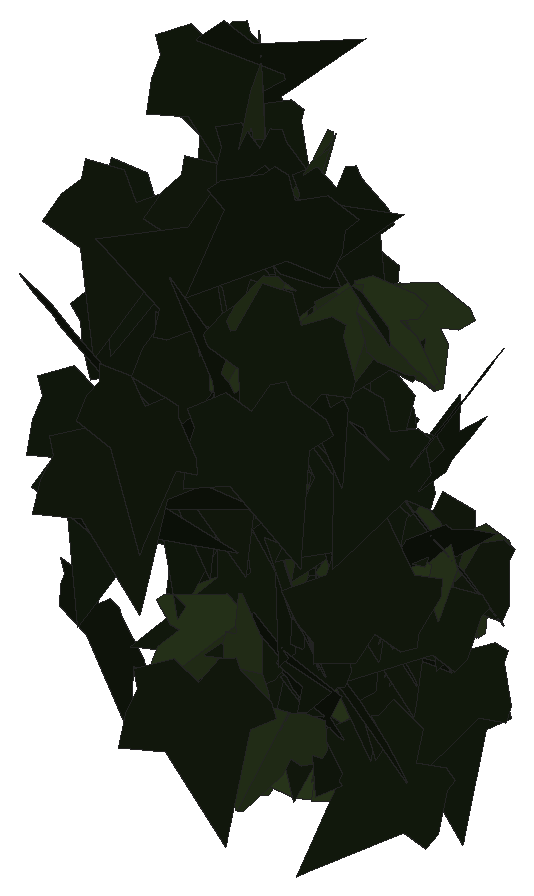
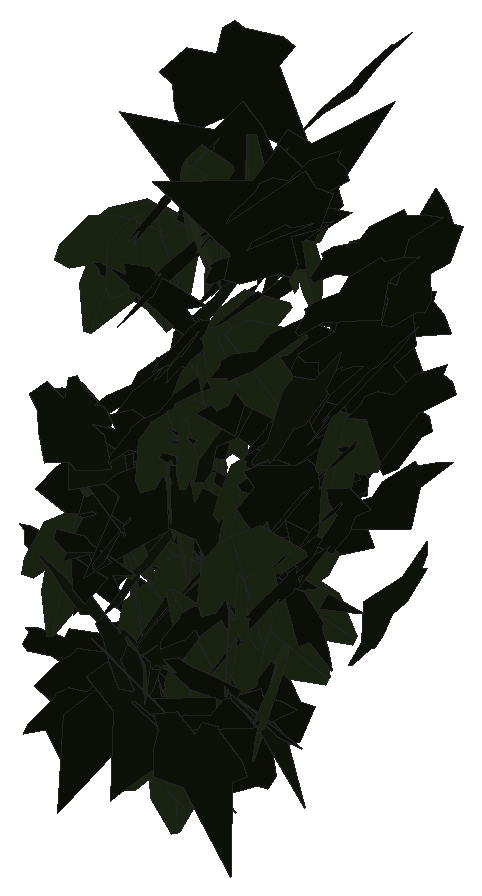
# SketchUp Ruby script. Lengths in inches.
U = 1.inch
M = Sketchup.active_model
def pt(a) = Geom::Point3d.new(a.map { |v| v * U })
def face(e, loops, mat)
  f = e.add_face(loops[0].map { |a| pt(a) })
  loops[1..].each { |l| e.add_face(l.map { |a| pt(a) }).erase! }
  f.material = f.back_material = mat if mat
  f
end
# faces: each face lists its corners as indices into pts; further lists are holes
def faces(e, pts, list, mat = nil) = list.each { |f| face(e, (f[0].is_a?(Array) ? f : [f]).map { |l| l.map { |i| pts[i] } }, mat) }
# xy, xz, yz: faces in a plane at the given z, y or x. An outline is a flat list of corners, or four numbers for a rectangle; further outlines are holes
def ring(l) = l.size == 4 ? [[l[0], l[1]], [l[2], l[1]], [l[2], l[3]], [l[0], l[3]]] : l.each_slice(2).to_a
def flat(e, list, mat, &to3) = list.each { |f| face(e, (f[0].is_a?(Array) ? f : [f]).map { |l| ring(l).map { |u, v| to3.(u, v) } }, mat) }
def xy(e, z, list, mat = nil) = flat(e, list, mat) { |x, y| [x, y, z] }
def xz(e, y, list, mat = nil) = flat(e, list, mat) { |x, z| [x, y, z] }
def yz(e, x, list, mat = nil) = flat(e, list, mat) { |y, z| [x, y, z] }
def lines(e, pts, list) = list.each { |a, b| e.add_line(pt(pts[a]), pt(pts[b])) }
# prism: a flat outline (further loops are holes) pulled along v
def prism(e, loops, v, mat = nil)
  f = face(e, loops, mat); d = Geom::Vector3d.new(v.map { |x| x * U })
  f.pushpull(f.normal.samedirection?(d) ? d.length : -d.length)
end
def box(e, o, s, mat = nil) = prism(e, [[o, [o[0] + s[0], o[1], o[2]], [o[0] + s[0], o[1] + s[1], o[2]], [o[0], o[1] + s[1], o[2]]]], [0, 0, s[2]], mat)
def at(x, y, z, deg = 0) = Geom::Transformation.translation(pt([x, y, z])) * Geom::Transformation.rotation(ORIGIN, Z_AXIS, deg.degrees)
def axes(o, x, y, z) = Geom::Transformation.new([*x, 0, *y, 0, *z, 0, *pt(o).to_a, 1])
def part(name) = M.definitions.add(name)
# library, detail: a bought-in or finely detailed component or shape, given as its bounding box
def library(name, o, s) = part(name).tap { |d| box(d.entities, o, s) }
def detail(e, o, s) = box(e.add_group.entities, o, s)
def put(e, d, t, mat = nil) = e.add_instance(d, t).tap { |i| i.material = mat if mat }
def group(e, t, mat = nil) = e.add_group.tap { |g| g.transformation = t; g.material = mat if mat }.entities
root = M.entities
M.materials.add("efeu1").color = [18, 25, 13]
M.materials.add("efeu2").color = [43, 57, 29]
c1 = part("ivyleaf_9")
p = [[1.54,2.16,1.25],[1.36,2.04,1.19],[-0.21,0.99,0.68],[-0.71,1.11,0.82],[-0.85,0.86,0.67],[-0.8,0.17,0.21],
  [-0.9,-0.01,0.1],[-0.67,-0.16,-0.02],[-0.08,-0.08,-0.05],[-0.03,-0.6,-0.4],[0.65,-0.88,-0.66],[0.83,-0.6,-0.49],
  [1.29,-0.42,-0.43],[1.8125,-0.07,-0.26],[1.21,0.44,0.15]]
faces(c1.entities,p,[[0,1,2,3,4,5,6,7,8,9,10,11,12,13,14]],"efeu1")
c2 = part("ivyleaf_10")
p = [[0,0.5,-0.03],[-0.0625,2.02,-0.43],[-0.19,2.01,-0.46],[-0.54,1.05,-0.29],[-0.52,0.625,-0.18],[-0.83,0.76,-0.28],
  [-1.16,0.64,-0.33],[-1.15,0.33,-0.24],[-0.77,-0.39,0.02],[-0.3,-0.51,0.16],[0.04,-0.48,0.23],[-0.02,2.01,-0.4375],
  [-0.06,2.01,-0.43],[0.04,-0.49,0.23],[0.67,-0.49,0.14],[1.38,0.36,-0.2],[1.375,0.51,-0.24],[0.81,0.65,-0.19],
  [0.62,0.59,-0.15],[0.6,1.09,-0.28],[0.5,1.23,-0.31]]
faces(c2.entities,p,[[0,1,2,3,4,5,6,7,8,9,10],[11,12,0,13,14,15,16,17,18,19,20]],"efeu2")
put(root,c1,axes([37.96,220.71,244.54],[-0.12354,-0.47923,0.07127],[-0.01994,-0.06846,-0.49489],[0.48409,-0.12511,-0.00219]))
put(root,c1,axes([37.8125,220.9,246.18],[0.24494,-0.40918,-0.15026],[-0.026,0.15834,-0.47355],[0.43512,0.2398,0.05629]))
put(root,c1,axes([37.8,222.26,246.11],[0.03675,-0.38064,0.32212],[0.1316,-0.30414,-0.37441],[0.48097,0.1123,0.07783]))
put(root,c1,axes([37.99,221.21,247.15],[-0.13138,-0.47417,0.08886],[-0.01747,-0.08736,-0.492],[0.48211,-0.13239,0.00639]))
put(root,c2,axes([38.11,221.03,245.32],[0.02039,-0.43408,-0.2473],[0.04694,0.24808,-0.43157],[0.49737,-0.00562,0.05087]))
put(root,c1,axes([37.83,220.61,243.18],[0.15949,-0.4167,0.22567],[0.09762,-0.20411,-0.44588],[0.46372,0.18628,0.01625]))
put(root,c1,axes([37.97,220.39,245.57],[-0.00115,-0.46441,-0.18526],[-0.01173,0.18524,-0.46427],[0.49986,0.00328,-0.01132]))
put(root,c2,axes([38.11,222.14,243.03],[-0.24291,0.43502,0.04189],[-0.01309,0.04066,-0.49817],[-0.43684,-0.24311,-0.00837]))
put(root,c1,axes([38,222.02,244.15],[0.27996,-0.29232,-0.29354],[-0.10891,0.28989,-0.39256],[0.3997,0.28374,0.09864]))
put(root,c1,axes([38.15,220.7,247.46],[-0.16154,-0.47243,0.02683],[-0.00693,-0.02598,-0.49928],[0.47314,-0.16167,0.00184]))
put(root,c1,axes([38.61,221.9,242.54],[-0.24635,0.39084,0.19118],[-0.11648,0.15244,-0.46173],[-0.41922,-0.27203,0.01594]))
put(root,c1,axes([38.21,221.57,244.29],[-0.00683,-0.48185,0.13332],[-0.00552,-0.13325,-0.48188],[0.49992,-0.00806,-0.0035]))
put(root,c1,axes([38.21,221.82,248.625],[0.01018,-0.46344,-0.18739],[-0.01552,0.18705,-0.46344],[0.49966,0.01525,-0.01058]))
put(root,c1,axes([38.6,222.85,242.4],[-0.16091,0.47337,-0.00515],[-0.01155,-0.00937,-0.49978],[-0.47326,-0.16072,0.01395]))
put(root,c2,axes([38.47,222.3125,244.32],[-0.20958,-0.43661,0.12428],[-0.0076,-0.13349,-0.48179],[0.45389,-0.20384,0.04932]))
put(root,c1,axes([38.2,221.38,244.9],[0.12038,-0.48516,0.01118],[0.0025,-0.01089,-0.49988],[0.48529,0.12041,-0.0002]))
put(root,c1,axes([38.13,221.5,244.9],[0.07711,-0.16743,-0.46478],[0.16347,0.45255,-0.13591],[0.46619,-0.131,0.12454]))
put(root,c1,axes([38.4,222.22,247.93],[-0.22111,-0.43508,0.10872],[0.00428,-0.12325,-0.48455],[0.44843,-0.21335,0.05823]))
put(root,c1,axes([38.1,222.01,248.16],[0.135,-0.04118,0.47967],[0.47348,0.10152,-0.12454],[-0.08714,0.48785,0.06641]))
put(root,c1,axes([38.1,219.6875,246.69],[0.26349,-0.28862,0.31188],[0.24141,-0.20034,-0.38934],[0.34971,0.35576,0.03378]))
put(root,c1,axes([38.6,220.89,245.02],[0.07759,0.49379,0.01219],[0.00013,0.01232,-0.49985],[-0.49394,0.07757,0.00179]))
put(root,c1,axes([38.36,221.5625,243.68],[-0.25895,-0.06159,-0.42326],[0.42123,0.04914,-0.26486],[0.07422,-0.49375,0.02643]))
put(root,c2,axes([38.54,222.28,243.87],[0.33302,-0.33002,-0.17374],[0.0094,0.24028,-0.43838],[0.37284,0.28871,0.16624]))
put(root,c1,axes([38.44,221.37,245.73],[0.0045,-0.49777,0.04695],[0.00857,-0.04687,-0.49772],[0.49991,0.00528,0.00811]))
put(root,c2,axes([38.66,221.54,243.07],[-0.08305,-0.34895,0.34834],[-0.00646,-0.35245,-0.3546],[0.49301,-0.0634,0.05403]))
put(root,c1,axes([38.45,221.42,245.01],[-0.04855,-0.43972,-0.23299],[0.05216,0.22831,-0.44176],[0.4949,-0.0672,0.02371]))
put(root,c1,axes([38.39,221.94,242],[0.02494,-0.02361,0.49882],[0.43276,0.25024,-0.00979],[-0.24919,0.43223,0.03292]))
put(root,c1,axes([38.96,222.61,242.92],[-0.48833,0.00779,0.10709],[-0.10733,-0.049,-0.48588],[0.00293,-0.49753,0.04953]))
put(root,c1,axes([38.625,222.54,242.52],[-0.19659,-0.45499,-0.06582],[0.01532,0.06506,-0.49551],[0.45948,-0.19684,-0.01164]))
put(root,c2,axes([38.8,221.7,248.63],[0.20938,-0.3969,-0.22054],[-0.01736,0.23568,-0.44063],[0.45372,0.19217,0.08491]))
put(root,c2,axes([38.78,221.83,244.86],[0.0064,-0.42454,-0.26406],[0.053,0.26317,-0.42182],[0.49714,-0.02259,0.04838]))
put(root,c2,axes([38.8,220.95,247.44],[0.16531,-0.47023,0.03944],[0.00288,-0.04079,-0.49833],[0.47187,0.16498,-0.01078]))
put(root,c1,axes([38.71,221.7,246.42],[-0.10637,-0.48741,-0.03343],[0.00489,0.03315,-0.49888],[0.48853,-0.10646,-0.00229]))
put(root,c2,axes([39.01,220.98,243.19],[-0.16994,-0.24865,0.39912],[-0.17326,-0.36141,-0.29894],[0.43715,-0.2399,0.03667]))
put(root,c2,axes([38.96,221.72,246.31],[-0.27625,-0.30282,0.28634],[-0.08549,-0.29505,-0.39451],[0.4079,-0.26692,0.11123]))
put(root,c1,axes([38.5,219.62,245],[0.42498,0.07261,0.25321],[0.24958,0.04275,-0.43114],[-0.08426,0.49285,0.0001]))
put(root,c1,axes([38.72,222.37,243.74],[-0.07377,-0.49231,-0.04683],[-0.00314,0.04781,-0.4977],[0.49452,-0.07314,-0.01014]))
put(root,c2,axes([38.74,222.29,242.84],[-0.36885,-0.1766,0.28769],[0.2826,0.07151,0.40623],[-0.18462,0.46228,0.04706]))
put(root,c1,axes([38.83,220.875,245.25],[0.16335,0.06778,0.46768],[0.24664,0.40986,-0.14554],[-0.4031,0.27825,0.10047]))
put(root,c1,axes([38.88,221.26,247.53],[-0.14764,-0.4776,0.0099],[-0.00315,-0.00939,-0.4999],[0.4777,-0.14767,-0.00024]))
put(root,c1,axes([39.19,221.96,244.69],[-0.19029,0.46185,0.02205],[-0.00887,0.02019,-0.49951],[-0.46229,-0.1905,0.00051]))
put(root,c2,axes([39.07,222.33,242.83],[-0.0141,-0.46427,0.18509],[0.00949,-0.18537,-0.46427],[0.49971,-0.00958,0.01404]))
put(root,c2,axes([39.08,221.64,246.53],[-0.05554,-0.46368,0.17864],[-0.0036,-0.17937,-0.4667],[0.49689,-0.05313,0.01658]))
put(root,c2,axes([39.11,221.63,244.47],[-0.49558,0.06051,0.02725],[-0.02746,-0.00005,-0.49925],[-0.06042,-0.49632,0.00337]))
put(root,c1,axes([39.39,221.33,243.45],[-0.40865,-0.07336,0.27861],[-0.27547,-0.04216,-0.41514],[0.0844,-0.49279,-0.00595]))
put(root,c1,axes([38.72,219.57,245.33],[0.36132,0.01669,0.34521],[0.34323,0.04116,-0.36125],[-0.04048,0.49802,0.01828]))
put(root,c2,axes([39.13,222.6,242.03],[-0.33719,-0.36551,0.05199],[0.05232,-0.11701,-0.48329],[0.36546,-0.32049,0.11715]))
put(root,c2,axes([39.06,222.49,241.9375],[0.00063,-0.20372,0.45662],[0.15138,-0.43511,-0.19433],[0.47653,0.13849,0.06112]))
put(root,c1,axes([39.25,222.65,242.57],[0.1329,0.41844,0.23926],[-0.01403,0.25144,-0.43195],[-0.48181,0.1081,0.07858]))
put(root,c1,axes([39.08,219.28,245.79],[-0.18011,-0.37787,-0.27344],[0.12041,0.24552,-0.4186],[0.45062,-0.21664,0.00256]))
put(root,c1,axes([39.49,222.72,242.29],[-0.49723,0.04762,0.02221],[-0.02225,0.00054,-0.4995],[-0.04759,-0.49773,0.00158]))
put(root,c2,axes([39.61,220.66,243.12],[-0.14071,0.08535,0.47214],[-0.46858,0.08128,-0.15435],[-0.1031,-0.48591,0.05711]))
put(root,c2,axes([39.08,221.51,241.98],[-0.06346,-0.15771,-0.47021],[0.31319,0.35483,-0.16127],[0.38456,-0.315,0.05375]))
put(root,c1,axes([39.04,221.24,246.75],[0.20052,-0.40808,-0.20799],[0.00025,0.22715,-0.44543],[0.45803,0.17853,0.0913]))
put(root,c1,axes([39.0625,221.44,248.02],[0.17718,-0.4667,-0.0282],[-0.01039,0.02622,-0.4992],[0.46744,0.17749,-0.0004]))
put(root,c2,axes([39.34,221.88,245.26],[0.04598,-0.49435,-0.05921],[-0.01432,0.05812,-0.4964],[0.49768,0.04735,-0.00882]))
put(root,c1,axes([39.4375,220.26,247.34],[-0.01755,0.015,0.49947],[-0.38324,-0.32111,-0.00382],[0.32065,-0.38297,0.02277]))
put(root,c2,axes([39.3125,222.27,244.87],[0.18484,-0.46087,-0.05864],[0.00327,0.0644,-0.49582],[0.46457,0.18291,0.02682]))
put(root,c1,axes([39.16,222.01,243.44],[-0.00539,-0.36133,0.34556],[0.02843,-0.34524,-0.36055],[0.49916,0.01576,0.02427]))
put(root,c1,axes([39.72,221.5,242.78],[-0.31089,0.26856,0.285],[-0.22972,0.16962,-0.41043],[-0.31714,-0.38614,0.01792]))
put(root,c2,axes([39.44,222.14,245.37],[-0.19502,-0.43799,0.14189],[-0.00097,-0.1537,-0.47579],[0.4604,-0.18585,0.0591]))
put(root,c1,axes([39.31,221.93,242.74],[-0.14978,-0.47421,-0.05183],[0.0107,0.05098,-0.49728],[0.47692,-0.15008,-0.00513]))
put(root,c1,axes([39.25,221.22,247.13],[-0.02145,-0.47988,0.13877],[0.01731,-0.13953,-0.47983],[0.49924,-0.01578,0.0226]))
put(root,c2,axes([39.54,221.55,245.7],[-0.05461,-0.44926,0.21256],[-0.02241,-0.21139,-0.45256],[0.4965,-0.05896,0.00295]))
put(root,c2,axes([39.47,221.8,247.92],[0.25745,-0.41902,0.09023],[0.03341,-0.08532,-0.49153],[0.42732,0.25912,-0.01594]))
put(root,c1,axes([39.84,222.65,242.8125],[-0.44897,0.20698,0.07474],[-0.08281,-0.00159,-0.49309],[-0.20388,-0.45515,0.03571]))
put(root,c1,axes([39.19,221.82,245.22],[0.20396,-0.34625,0.29751],[0.23964,-0.19615,-0.39256],[0.38856,0.30272,0.08593]))
put(root,c1,axes([39.83,222.49,242.99],[-0.34022,0.36251,-0.05326],[0.0411,-0.03446,-0.49711],[-0.36409,-0.34263,-0.00636]))
put(root,c1,axes([39.31,222.53,242.95],[0.02599,-0.28604,0.40927],[0.23612,-0.35407,-0.26245],[0.43997,0.20691,0.11668]))
put(root,c2,axes([39.64,221.55,248.02],[0.13789,-0.47936,0.03459],[0.00452,-0.03469,-0.49877],[0.48059,0.13786,-0.00524]))
put(root,c1,axes([39.44,222.11,244.83],[0.02766,-0.21724,-0.44949],[0.02348,0.45025,-0.21616],[0.49868,-0.00915,0.03511]))
put(root,c1,axes([39.55,219.91,243.24],[-0.1136,-0.42264,-0.24181],[0.06184,0.23378,-0.43764],[0.48298,-0.12934,-0.00084]))
put(root,c2,axes([39.66,221.46,241.74],[0.30332,0.3785,-0.12138],[0.07387,0.09636,0.48504],[0.39056,-0.31218,0.00254]))
put(root,c2,axes([39.61,222.62,242.67],[-0.34873,0.28021,-0.22332],[0.14591,-0.17356,-0.44563],[-0.32726,-0.37598,0.03928]))
put(root,c2,axes([39.88,220.68,242.6],[-0.28797,-0.36641,0.18114],[-0.12022,-0.13586,-0.46593],[0.39067,-0.3119,-0.00985]))
put(root,c2,axes([39.8,221.99,243.33],[0.12952,0.4081,-0.25822],[-0.17497,-0.20953,-0.41891],[-0.45012,0.19888,0.08854]))
put(root,c2,axes([39.75,222.46,242.64],[0.2757,-0.3919,-0.14284],[0.00303,0.1731,-0.46907],[0.41711,0.25778,0.09782]))
put(root,c1,axes([39.84,220.07,246.31],[0.16086,-0.43233,0.19291],[-0.02603,0.19536,0.45952],[-0.4727,-0.15788,0.04034]))
put(root,c2,axes([39.81,220.69,246.99],[0.06862,0.34856,-0.35185],[-0.14786,-0.3246,-0.35039],[-0.47268,0.15214,0.05853]))
put(root,c1,axes([39.5625,221.46,247.375],[0.27395,-0.31436,-0.27592],[-0.06589,0.29328,-0.39956],[0.41305,0.25528,0.11926]))
put(root,c1,axes([39.625,222.15,245.58],[0.01672,-0.4997,0.00498],[-0.00584,-0.00518,-0.49994],[0.49969,0.01666,-0.00601]))
put(root,c1,axes([39.76,221.52,245.38],[0.42998,0.14103,-0.21266],[-0.20488,-0.05759,-0.45244],[-0.15211,0.47623,0.00826]))
put(root,c2,axes([39.83,221.91,242.11],[0.06883,-0.49116,-0.06344],[-0.00242,0.06372,-0.49592],[0.49523,0.06857,0.00639]))
put(root,c1,axes([39.6,222.5,243.875],[0.02038,-0.39437,0.30668],[0.06832,-0.30185,-0.3927],[0.49489,0.05791,0.04159]))
put(root,c1,axes([39.84,222.12,244.82],[-0.24684,-0.40581,0.15616],[-0.05281,-0.15026,-0.47396],[0.4316,-0.25048,0.03131]))
put(root,c1,axes([39.65,221.3,246.25],[0.12972,-0.45072,-0.17327],[-0.03994,0.16878,-0.46895],[0.48123,0.13551,0.00779]))
put(root,c2,axes([39.87,220.93,244.0625],[-0.2967,0.39444,0.07988],[-0.05214,0.06073,-0.49355],[-0.39906,-0.30121,0.00509]))
put(root,c1,axes([39.53,221.27,242.76],[0.00922,-0.18967,0.46254],[0.31086,-0.36012,-0.15387],[0.39151,0.29041,0.11128]))
put(root,c1,axes([39.64,221.875,243.25],[0.14674,-0.47709,0.02922],[0.01095,-0.02721,-0.49914],[0.47786,0.14712,0.00246]))
put(root,c1,axes([39.72,221.97,242.1],[-0.12568,-0.35642,0.32736],[0.10145,-0.35011,-0.34224],[0.4732,-0.01961,0.16032]))
put(root,c1,axes([40.14,222.14,245.17],[-0.47695,-0.13296,0.06961],[-0.06893,-0.01195,-0.49508],[0.13331,-0.48185,-0.00693]))
put(root,c1,axes([40.03,222,244.53],[-0.41555,-0.2677,-0.07521],[0.05499,0.05346,-0.49408],[0.27258,-0.4189,-0.01499]))
put(root,c1,axes([39.72,221.375,246.23],[0.15292,-0.45106,0.15218],[0.06816,-0.13745,-0.47588],[0.47114,0.16628,0.01945]))
put(root,c1,axes([39.79,222.34,242.74],[-0.03892,-0.44839,0.21779],[0.12369,-0.2203,-0.43147],[0.48289,0.02029,0.12807]))
put(root,c1,axes([39.95,222.5,242.45],[0.43859,0.19029,-0.1464],[-0.1401,-0.04475,-0.47788],[-0.19497,0.4602,0.01406]))
put(root,c1,axes([40.05,221.85,244.69],[-0.24328,-0.29715,0.32019],[-0.06607,-0.33725,-0.36318],[0.4318,-0.21902,0.12483]))
put(root,c1,axes([40.4,220.99,243.52],[-0.31732,0.31233,0.22751],[-0.18321,0.13759,-0.44441],[-0.34021,-0.36541,0.02712]))
put(root,c1,axes([39.67,220.8125,247.62],[0.08703,-0.04141,0.49062],[0.47981,-0.10467,-0.09395],[0.11048,0.48717,0.02152]))
put(root,c1,axes([39.8,221.84,244.04],[0.30123,-0.39907,0.00244],[-0.0004,-0.00336,-0.49999],[0.39908,0.30122,-0.00234]))
put(root,c2,axes([40.08,222.08,243.6],[0.29961,-0.39857,-0.03706],[0.00486,0.04991,-0.49748],[0.40026,0.29774,0.03378]))
put(root,c1,axes([39.78,221.49,243.03],[0.34883,-0.33811,0.11832],[0.08525,-0.08206,-0.4858],[0.34793,0.35909,0.0004]))
put(root,c1,axes([39.92,221.5,247.87],[0.20293,-0.45089,-0.07429],[-0.02371,0.07079,-0.4944],[0.45635,0.20418,0.00735]))
put(root,c2,axes([40.32,221.71,243.98],[0.27863,0.28788,-0.29916],[-0.27391,-0.14329,-0.39299],[-0.312,0.38288,0.07786]))
put(root,c1,axes([40.33,221.76,246.75],[-0.4809,-0.12808,-0.04832],[0.05269,-0.01029,-0.49711],[0.12635,-0.48321,0.0234]))
put(root,c1,axes([40.1875,220.57,246.9375],[-0.28061,-0.41321,-0.02279],[0.01512,0.01729,-0.49947],[0.41356,-0.281,0.00279]))
put(root,c1,axes([40.46,220.13,248.5625],[0.04692,0.17453,-0.4662],[-0.16609,-0.43594,-0.17992],[-0.46927,0.17175,0.01706]))
put(root,c2,axes([40.54,222.03,244.17],[0.31667,-0.10286,-0.37302],[-0.34681,0.13831,-0.33256],[0.17159,0.46935,0.01625]))
put(root,c1,axes([40.14,221.84,243.96],[-0.00916,-0.46801,-0.17574],[0.03931,0.17455,-0.46689],[0.49837,-0.02237,0.03359]))
put(root,c1,axes([40.19,222.64,242.29],[-0.03705,-0.46669,-0.17559],[0.00744,0.17554,-0.46811],[0.49857,-0.0373,-0.00606]))
put(root,c1,axes([40.57,222.5,245.49],[-0.26157,0.40999,-0.11616],[0.05219,-0.10445,-0.48618],[-0.42292,-0.26646,0.01184]))
put(root,c2,axes([40.46,221.38,246.96],[-0.18261,-0.44845,0.1247],[-0.02712,-0.12348,-0.48375],[0.46467,-0.18344,0.02077]))
put(root,c1,axes([40.51,221.87,244.89],[0.16627,0.31344,0.35229],[-0.10279,0.38866,-0.29728],[-0.4602,0.02643,0.19369]))
put(root,c1,axes([40.13,222.25,244.42],[0.44602,-0.22597,0.00145],[0.00065,-0.00191,-0.5],[0.22597,0.44602,-0.00141]))
put(root,c1,axes([40.68,222.46,243.5],[-0.43128,0.2521,-0.02104],[-0.00449,-0.04922,-0.49755],[-0.25293,-0.42898,0.04472]))
put(root,c1,axes([40.38,221.64,245.43],[-0.149,-0.4512,0.15562],[-0.01087,-0.15978,-0.47366],[0.47716,-0.14453,0.03781]))
put(root,c1,axes([40.52,222.55,242.77],[-0.40698,-0.27136,-0.10358],[0.12152,0.00286,-0.485],[0.26381,-0.41995,0.06362]))
put(root,c1,axes([40.52,221.67,244.21],[0.2258,0.44455,0.03733],[-0.00612,0.04492,-0.49794],[-0.44607,0.22441,0.02573]))
put(root,c1,axes([40.61,222.59,243.91],[-0.46281,-0.15921,-0.10225],[0.1082,-0.00103,-0.48815],[0.15523,-0.47397,0.0354]))
put(root,c1,axes([40.75,222.04,243.77],[-0.46109,-0.16493,0.10099],[-0.07387,-0.09109,-0.48605],[0.17872,-0.46314,0.05963]))
put(root,c2,axes([40.37,221.22,246.97],[-0.38169,-0.04142,-0.32031],[0.31643,0.05144,-0.3837],[0.06474,-0.49562,-0.01306]))
put(root,c2,axes([40.57,222.41,243.87],[-0.20009,-0.43686,-0.13826],[0.0904,0.11026,-0.47924],[0.44921,-0.21678,0.03486]))
put(root,c1,axes([40.79,221.47,242.18],[-0.46441,-0.17483,0.06133],[-0.05865,-0.01826,-0.49621],[0.17575,-0.46808,-0.00354]))
put(root,c1,axes([40.75,220.97,243.85],[-0.39561,-0.21056,0.22172],[0.19368,0.10799,0.44814],[-0.23661,0.44046,-0.00388]))
put(root,c1,axes([40.49,219.54,246.58],[-0.05357,-0.40415,-0.28947],[0.03869,0.28688,-0.40768],[0.49561,-0.06608,0.00054]))
put(root,c1,axes([40.46,217.98,247.32],[0.01648,-0.4832,0.12748],[0.0373,-0.126,-0.48242],[0.49833,0.02541,0.03189]))
put(root,c2,axes([40.65,221.54,246.95],[-0.43277,-0.22104,-0.11767],[0.10924,0.04477,-0.48586],[0.22533,-0.44625,0.00955]))
